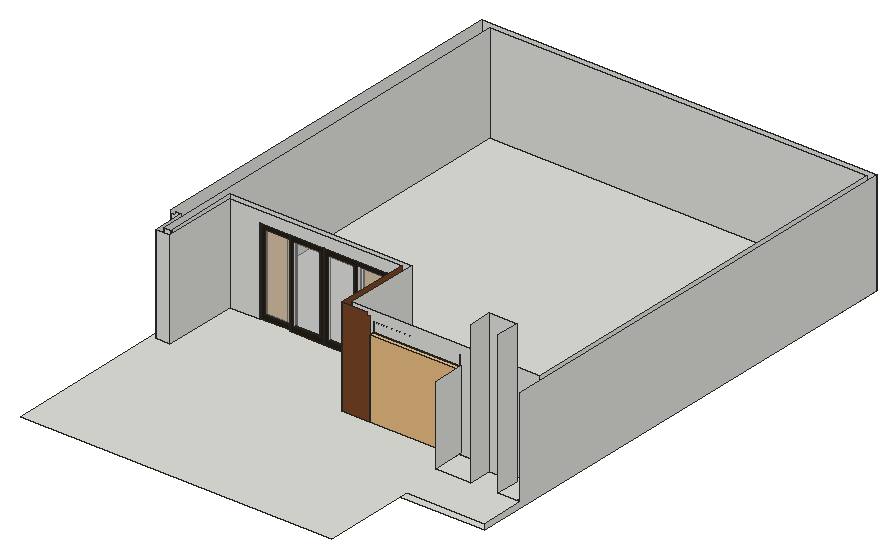
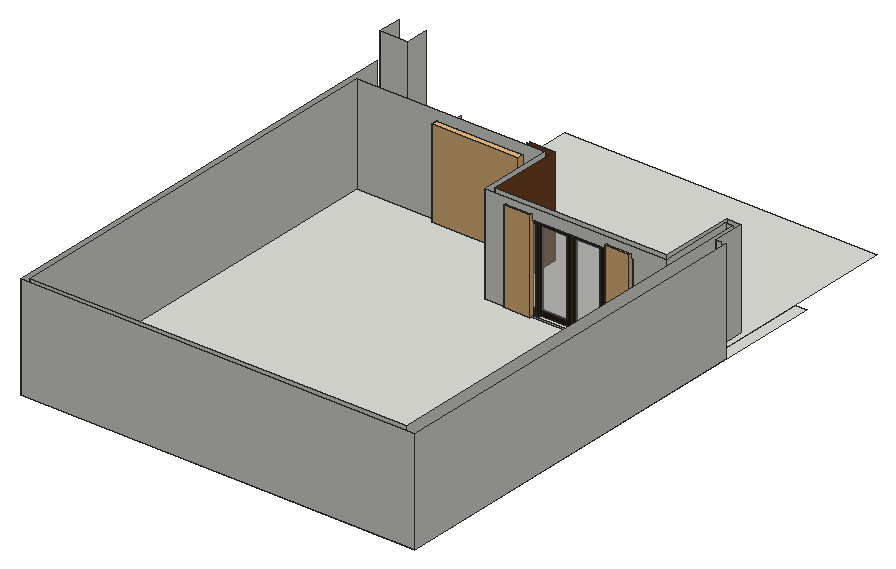
# SketchUp Ruby script. Lengths in inches.
U = 1.inch
M = Sketchup.active_model
def pt(a) = Geom::Point3d.new(a.map { |v| v * U })
def face(e, loops, mat)
  f = e.add_face(loops[0].map { |a| pt(a) })
  loops[1..].each { |l| e.add_face(l.map { |a| pt(a) }).erase! }
  f.material = f.back_material = mat if mat
  f
end
# faces: each face lists its corners as indices into pts; further lists are holes
def faces(e, pts, list, mat = nil) = list.each { |f| face(e, (f[0].is_a?(Array) ? f : [f]).map { |l| l.map { |i| pts[i] } }, mat) }
# xy, xz, yz: faces in a plane at the given z, y or x. An outline is a flat list of corners, or four numbers for a rectangle; further outlines are holes
def ring(l) = l.size == 4 ? [[l[0], l[1]], [l[2], l[1]], [l[2], l[3]], [l[0], l[3]]] : l.each_slice(2).to_a
def flat(e, list, mat, &to3) = list.each { |f| face(e, (f[0].is_a?(Array) ? f : [f]).map { |l| ring(l).map { |u, v| to3.(u, v) } }, mat) }
def xy(e, z, list, mat = nil) = flat(e, list, mat) { |x, y| [x, y, z] }
def xz(e, y, list, mat = nil) = flat(e, list, mat) { |x, z| [x, y, z] }
def yz(e, x, list, mat = nil) = flat(e, list, mat) { |y, z| [x, y, z] }
def lines(e, pts, list) = list.each { |a, b| e.add_line(pt(pts[a]), pt(pts[b])) }
# prism: a flat outline (further loops are holes) pulled along v
def prism(e, loops, v, mat = nil)
  f = face(e, loops, mat); d = Geom::Vector3d.new(v.map { |x| x * U })
  f.pushpull(f.normal.samedirection?(d) ? d.length : -d.length)
end
def box(e, o, s, mat = nil) = prism(e, [[o, [o[0] + s[0], o[1], o[2]], [o[0] + s[0], o[1] + s[1], o[2]], [o[0], o[1] + s[1], o[2]]]], [0, 0, s[2]], mat)
def at(x, y, z, deg = 0) = Geom::Transformation.translation(pt([x, y, z])) * Geom::Transformation.rotation(ORIGIN, Z_AXIS, deg.degrees)
def axes(o, x, y, z) = Geom::Transformation.new([*x, 0, *y, 0, *z, 0, *pt(o).to_a, 1])
def part(name) = M.definitions.add(name)
# library, detail: a bought-in or finely detailed component or shape, given as its bounding box
def library(name, o, s) = part(name).tap { |d| box(d.entities, o, s) }
def detail(e, o, s) = box(e.add_group.entities, o, s)
def put(e, d, t, mat = nil) = e.add_instance(d, t).tap { |i| i.material = mat if mat }
def group(e, t, mat = nil) = e.add_group.tap { |g| g.transformation = t; g.material = mat if mat }.entities
root = M.entities
M.materials.add("[Translucent Glass Gray]2").color = [201, 201, 201]
M.materials["[Translucent Glass Gray]2"].alpha = 0.5
M.materials.add("[Wood Veneer 01]").color = [120, 70, 37]
M.materials.add("curtain").color = [207, 207, 207]
M.materials["curtain"].alpha = 0.74
M.materials.add("oak swatch").color = [40, 31, 19]
c1 = library("Sliding Door",[0,0,0],[94.49,5.83,91.73])
c2 = library("Window curtains",[0,0,0],[5.91,79.92,51.3])
c3 = part("Group\#1")
box(c3.entities,[0,0,0],[1.77,4.72,80.31],"oak swatch")
c4 = part("Exterior Sliding Doors")
xy(c4.entities,0,[[1.77,33.07,3.54,70.87],[1.77,70.87,3.54,108.66]])
xy(c4.entities,0,[[0,0,1.77,33.07],[0,108.66,1.77,141.73]],"oak swatch")
xy(c4.entities,4.72,[[0,4.72,1.77,33.07],[1.77,37.8,3.54,66.14],[1.77,75.88,3.54,103.9375],[0,108.66,1.77,137.01]],"oak swatch")
xy(c4.entities,75.59,[[1.77,37.8,3.54,66.14],[1.77,75.88,3.54,103.9375]])
xy(c4.entities,75.59,[[0,4.72,1.77,33.07],[0,108.66,1.77,137.01]],"oak swatch")
xy(c4.entities,80.31,[[0,0,1.77,33.07],[1.77,33.07,3.54,70.87],[1.77,70.87,3.54,108.66],[0,108.66,1.77,141.73]],"oak swatch")
xz(c4.entities,0,[[0,0,1.77,80.31]],"oak swatch")
xz(c4.entities,4.72,[[0,4.72,1.77,75.59]],"oak swatch")
xz(c4.entities,33.07,[[0,0,1.77,4.72],[1.77,0,3.54,80.31],[0,75.59,1.77,80.31]],"oak swatch")
xz(c4.entities,37.8,[[1.77,4.72,3.54,75.59]])
xz(c4.entities,66.14,[[1.77,4.72,3.54,75.59]],"oak swatch")
xz(c4.entities,70.87,[[1.77,0,3.54,80.31]])
xz(c4.entities,75.88,[[1.77,4.72,3.54,75.59]])
xz(c4.entities,103.9375,[[1.77,4.72,3.54,75.59]],"oak swatch")
xz(c4.entities,108.66,[[1.77,4.72,3.54,75.59]])
xz(c4.entities,108.66,[[0,0,3.54,4.72],[0,75.59,3.54,80.31]],"oak swatch")
xz(c4.entities,137.01,[[0,4.72,1.77,75.59]],"oak swatch")
xz(c4.entities,141.73,[[0,0,1.77,80.31]],"oak swatch")
yz(c4.entities,0,[[0,0,33.07,0,33.07,4.72,4.72,4.72,4.72,75.59,33.07,75.59,33.07,80.31,0,80.31],[108.66,0,141.73,0,141.73,80.31,108.66,80.31,108.66,75.59,137.01,75.59,137.01,4.72,108.66,4.72]],"oak swatch")
yz(c4.entities,1.77,[[4.72,4.72,33.07,75.59],[37.8,4.72,66.14,75.59],[75.88,4.72,103.9375,75.59],[108.66,4.72,137.01,75.59]],"[Translucent Glass Gray]2")
yz(c4.entities,1.77,[[0,0,33.07,0,33.07,4.72,4.72,4.72,4.72,75.59,33.07,75.59,33.07,80.31,0,80.31],[[33.07,0,70.87,80.31],[37.8,4.72,66.14,75.59]],[[70.87,0,141.73,80.31],[108.66,4.72,137.01,75.59],[75.88,4.72,103.9375,75.59]]],"oak swatch")
yz(c4.entities,3.54,[[[33.07,0,70.87,80.31],[37.8,4.72,66.14,75.59]],[[70.87,0,108.66,80.31],[75.88,4.72,103.9375,75.59]]],"oak swatch")
put(c4.entities,c3,at(0,33.07,0))
put(c4.entities,c3,at(0,103.9375,0))
c5 = library("Plane02",[0.84,-3.92,-95.52],[32.2,7.84,95.63])
xy(root,252,[[177.75,508.37,177.75,1103.3125,657.75,1103.3125,657.75,508.37,431.89,508.37,431.89,692.93,220.5,692.93,220.5,721.37,447.875,721.37,447.875,522.1,645.31,522.1,645.31,1090.87,190.19,1090.87,190.19,508.37],[190.19,508.37,190.19,721.37,220.5,721.37,220.5,692.93,220.4375,692.93,220.4375,508.37],[[447.875,522.1,447.875,721.37,190.19,721.37,190.19,1090.87,645.31,1090.87,645.31,522.1],[380.99,855.03,382.54,855.24,383.99,855.84,385.23,856.79,386.1875,858.03,386.79,859.48,386.99,861.03,386.79,862.59,386.1875,864.03,385.23,865.28,383.99,866.23,382.54,866.83,380.99,867.03,379.4375,866.83,377.99,866.23,376.75,865.28,375.8,864.03,375.2,862.59,374.99,861.03,375.2,859.48,375.8,858.03,376.75,856.79,377.99,855.84,379.4375,855.24],[312.79,972.48,314.35,972.6875,315.79,973.29,317.04,974.24,317.99,975.48,318.59,976.93,318.79,978.48,318.59,980.04,317.99,981.48,317.04,982.72,315.79,983.68,314.35,984.28,312.79,984.48,311.24,984.28,309.79,983.68,308.55,982.72,307.6,981.48,307,980.04,306.79,978.48,307,976.93,307.6,975.48,308.55,974.24,309.79,973.29,311.24,972.6875],[380.99,920.01,382.54,920.22,383.99,920.81,385.23,921.77,386.1875,923.01,386.79,924.46,386.99,926.01,386.79,927.5625,386.1875,929.01,385.23,930.25,383.99,931.21,382.54,931.81,380.99,932.01,379.4375,931.81,377.99,931.21,376.75,930.25,375.8,929.01,375.2,927.5625,374.99,926.01,375.2,924.46,375.8,923.01,376.75,921.77,377.99,920.81,379.4375,920.22],[380.99,982.21,382.54,982.41,383.99,983.01,385.23,983.97,386.1875,985.21,386.79,986.66,386.99,988.21,386.79,989.76,386.1875,991.21,385.23,992.45,383.99,993.41,382.54,994.01,380.99,994.21,379.4375,994.01,377.99,993.41,376.75,992.45,375.8,991.21,375.2,989.76,374.99,988.21,375.2,986.66,375.8,985.21,376.75,983.97,377.99,983.01,379.4375,982.41],[312.79,900.05,314.04,900.21,315.2,900.7,316.2,901.46,316.97,902.46,317.45,903.62,317.61,904.87,317.45,906.11,316.97,907.28,316.2,908.27,315.2,909.04,314.04,909.52,312.79,909.68,311.55,909.52,310.39,909.04,309.39,908.27,308.62,907.28,308.14,906.11,307.98,904.87,308.14,903.62,308.62,902.46,309.39,901.46,310.39,900.7,311.55,900.21],[312.79,849.57,313.47,849.66,314.11,849.93,314.65,850.34,315.07,850.89,315.33,851.52,315.42,852.2,315.33,852.88,315.07,853.51,314.65,854.05,314.11,854.47,313.47,854.73,312.79,854.82,312.12,854.73,311.48,854.47,310.9375,854.05,310.52,853.51,310.26,852.88,310.17,852.2,310.26,851.52,310.52,850.89,310.9375,850.34,311.48,849.93,312.12,849.66]],[447.875,707.71,645.31,721.37]])
xy(root,253.1875,[[236.74,560.96,235.44,561.13,234.24,561.625,233.2,562.42,232.4,563.46,231.91,564.66,231.74,565.96,231.91,567.25,232.4,568.46,233.2,569.49,234.24,570.29,235.44,570.79,236.74,570.96,238.03,570.79,239.24,570.29,240.27,569.49,241.07,568.46,241.56,567.25,241.74,565.96,241.56,564.66,241.07,563.46,240.27,562.42,239.24,561.625,238.03,561.13]])
xy(root,258,[[193.12,600.32,201.88,600.32,201.88,690.57,422.81,690.57,422.81,600.32,651,600.32,651,1096.57,193.12,1096.57]])
xy(root,259.4375,[[183.75,394.64,562.6875,394.64,562.6875,508.37,657.75,508.37,657.75,562.125,631.02,562.125,631.02,589.625,597.99,589.625,597.99,562.125,554.88,562.125,554.88,600.32,449.19,600.32,449.19,593.57,416.0625,593.57,416.0625,683.82,398.4,683.82,398.4,690.57,243.65,690.57,243.65,683.82,206.9375,683.82,206.9375,593.57,189.75,593.57,189.75,631.27,183.75,631.27]])
xz(root,589.625,[[597.99,259.4375,631.02,431.7]])
xz(root,593.57,[[189.75,259.4375,206.9375,378]])
xz(root,593.57,[[416.0625,259.4375,449.19,259.4375,449.19,354.1875,449.43,354.1875,449.43,375.25,446,375.25,446,378,416.0625,378]],"[Wood Veneer 01]")
xz(root,600.32,[[193.12,258,201.88,378],[201.88,258,202.875,378],[422.81,258,422.81,378,651,378,651,258,554.88,258,554.88,354.1875,449.19,354.1875,449.19,258],[449.19,258,554.88,259.4375]])
xz(root,631.27,[[183.75,259.4375,189.75,259.4375,189.75,378,183.75,378,183.75,375.25,177.75,375.25,177.75,273.1875,183.75,273.1875]])
xz(root,683.82,[[206.9375,259.4375,243.65,259.4375,243.65,364.125,398.4,364.125,398.4,259.4375,416.0625,259.4375,416.0625,378,206.9375,378]])
xz(root,690.57,[[201.88,258,201.88,378,422.81,378,422.81,258,398.4,258,398.4,364.125,243.65,364.125,243.65,258],[243.65,258,398.4,259.4375]])
xz(root,1096.57,[[193.12,258,651,378]])
xz(root,1103.3125,[[177.75,252,657.75,378]])
yz(root,177.75,[[631.27,252,1103.3125,378]])
yz(root,189.75,[[593.57,259.4375,631.27,378]])
yz(root,193.12,[[600.32,258,1096.57,378]])
yz(root,201.88,[[600.32,258,690.57,378]])
yz(root,206.9375,[[593.57,259.4375,683.82,378]])
yz(root,243.65,[[683.82,259.4375,690.57,364.125]])
yz(root,398.4,[[683.82,259.4375,690.57,364.125]])
yz(root,416.0625,[[593.57,259.4375,683.82,378]],"[Wood Veneer 01]")
yz(root,422.81,[[600.32,258,690.57,378]])
yz(root,449.19,[[593.57,259.4375,600.32,354.1875]])
yz(root,554.88,[[562.125,259.4375,600.32,354.1875]])
yz(root,597.99,[[562.125,259.4375,589.625,431.7]])
yz(root,631.02,[[562.125,259.4375,589.625,431.7]])
yz(root,651,[[600.32,258,1096.57,378]])
yz(root,657.75,[[508.37,252,1103.3125,252,1103.3125,378,562.125,378,562.125,259.4375,508.37,259.4375]])
p = [[231.74,565.96,252],[231.91,567.25,252],[231.91,567.25,253.1875],[231.74,565.96,253.1875],[241.56,567.25,252],[241.74,565.96,252],
  [241.74,565.96,253.1875],[241.56,567.25,253.1875],[282.24,565.96,252],[282.41,567.25,252],[282.41,567.25,253.1875],[282.24,565.96,253.1875],
  [292.06,567.25,252],[292.24,565.96,252],[292.24,565.96,253.1875],[292.06,567.25,253.1875],[332.74,565.96,252],[332.91,567.25,252],
  [332.91,567.25,253.1875],[332.74,565.96,253.1875],[342.56,567.25,252],[342.74,565.96,252],[342.74,565.96,253.1875],[342.56,567.25,253.1875],
  [383.24,565.96,252],[383.41,567.25,252],[383.41,567.25,253.1875],[383.24,565.96,253.1875],[393.06,567.25,252],[393.24,565.96,252],
  [393.24,565.96,253.1875],[393.06,567.25,253.1875],[232.4,568.46,252],[232.4,568.46,253.1875],[241.07,568.46,252],[241.07,568.46,253.1875],
  [282.9,568.46,252],[282.9,568.46,253.1875],[291.57,568.46,252],[291.57,568.46,253.1875],[333.4,568.46,252],[333.4,568.46,253.1875],
  [342.07,568.46,252],[342.07,568.46,253.1875],[383.9,568.46,252],[383.9,568.46,253.1875],[392.57,568.46,252],[392.57,568.46,253.1875],
  [233.2,569.49,252],[233.2,569.49,253.1875],[240.27,569.49,252],[240.27,569.49,253.1875],[283.7,569.49,252],[283.7,569.49,253.1875],
  [290.77,569.49,252],[290.77,569.49,253.1875],[334.2,569.49,252],[334.2,569.49,253.1875],[341.27,569.49,252],[341.27,569.49,253.1875],
  [384.7,569.49,252],[384.7,569.49,253.1875],[391.77,569.49,252],[391.77,569.49,253.1875],[234.24,570.29,252],[234.24,570.29,253.1875],
  [239.24,570.29,252],[239.24,570.29,253.1875],[284.74,570.29,252],[284.74,570.29,253.1875],[289.74,570.29,252],[289.74,570.29,253.1875],
  [335.24,570.29,252],[335.24,570.29,253.1875],[340.24,570.29,252],[340.24,570.29,253.1875],[385.74,570.29,252],[385.74,570.29,253.1875],
  [390.74,570.29,252],[390.74,570.29,253.1875],[235.44,570.79,252],[235.44,570.79,253.1875],[238.03,570.79,252],[238.03,570.79,253.1875],
  [285.94,570.79,252],[285.94,570.79,253.1875],[288.53,570.79,252],[288.53,570.79,253.1875],[336.44,570.79,252],[336.44,570.79,253.1875],
  [339.03,570.79,252],[339.03,570.79,253.1875],[386.94,570.79,252],[386.94,570.79,253.1875],[389.53,570.79,252],[389.53,570.79,253.1875],
  [236.74,570.96,252],[236.74,570.96,253.1875],[287.24,570.96,252],[287.24,570.96,253.1875],[337.74,570.96,252],[337.74,570.96,253.1875],
  [388.24,570.96,252],[388.24,570.96,253.1875],[312.79,849.57,252],[312.12,849.66,252],[312.12,849.66,252.625],[312.79,849.57,252.625],
  [313.47,849.66,252],[313.47,849.66,252.625],[311.48,849.93,252],[311.48,849.93,252.625],[314.11,849.93,252],[314.11,849.93,252.625],
  [310.9375,850.34,252],[310.9375,850.34,252.625],[314.65,850.34,252],[314.65,850.34,252.625],[310.52,850.89,252],[310.52,850.89,252.625],
  [315.07,850.89,252],[315.07,850.89,252.625],[310.26,851.52,252],[310.26,851.52,252.625],[315.33,851.52,252],[315.33,851.52,252.625],
  [310.17,852.2,252],[310.17,852.2,252.625],[315.42,852.2,252],[315.42,852.2,252.625],[310.26,852.88,252],[310.26,852.88,252.625],
  [315.33,852.88,252],[315.33,852.88,252.625],[310.52,853.51,252],[310.52,853.51,252.625],[315.07,853.51,252],[315.07,853.51,252.625],
  [310.9375,854.05,252],[310.9375,854.05,252.625],[314.65,854.05,252],[314.65,854.05,252.625],[311.48,854.47,252],[311.48,854.47,252.625],
  [314.11,854.47,252],[314.11,854.47,252.625],[312.12,854.73,252],[312.12,854.73,252.625],[313.47,854.73,252],[313.47,854.73,252.625],
  [312.79,854.82,252],[312.79,854.82,252.625],[380.99,855.03,252],[379.4375,855.24,252],[379.4375,855.24,253.3125],[380.99,855.03,253.3125],
  [382.54,855.24,252],[382.54,855.24,253.3125],[377.99,855.84,252],[377.99,855.84,253.3125],[383.99,855.84,252],[383.99,855.84,253.3125],
  [376.75,856.79,252],[376.75,856.79,253.3125],[385.23,856.79,252],[385.23,856.79,253.3125],[375.8,858.03,252],[375.8,858.03,253.3125],
  [386.1875,858.03,252],[386.1875,858.03,253.3125],[375.2,859.48,252],[375.2,859.48,253.3125],[386.79,859.48,252],[386.79,859.48,253.3125],
  [374.99,861.03,252],[374.99,861.03,253.3125],[386.99,861.03,252],[386.99,861.03,253.3125],[375.2,862.59,252],[375.2,862.59,253.3125],
  [386.79,862.59,252],[386.79,862.59,253.3125],[375.8,864.03,252],[375.8,864.03,253.3125],[386.1875,864.03,252],[386.1875,864.03,253.3125],
  [376.75,865.28,252],[376.75,865.28,253.3125],[385.23,865.28,252],[385.23,865.28,253.3125],[377.99,866.23,252],[377.99,866.23,253.3125],
  [383.99,866.23,252],[383.99,866.23,253.3125],[379.4375,866.83,252],[379.4375,866.83,253.3125],[382.54,866.83,252],[382.54,866.83,253.3125],
  [380.99,867.03,252],[380.99,867.03,253.3125],[312.79,900.05,252],[311.55,900.21,252],[311.55,900.21,252.625],[312.79,900.05,252.625],
  [314.04,900.21,252],[314.04,900.21,252.625],[310.39,900.7,252],[310.39,900.7,252.625],[315.2,900.7,252],[315.2,900.7,252.625],
  [309.39,901.46,252],[309.39,901.46,252.625],[316.2,901.46,252],[316.2,901.46,252.625],[308.62,902.46,252],[308.62,902.46,252.625],
  [316.97,902.46,252],[316.97,902.46,252.625],[308.14,903.62,252],[308.14,903.62,252.625],[317.45,903.62,252],[317.45,903.62,252.625],
  [307.98,904.87,252],[307.98,904.87,252.625],[317.61,904.87,252],[317.61,904.87,252.625],[308.14,906.11,252],[308.14,906.11,252.625],
  [317.45,906.11,252],[317.45,906.11,252.625],[308.62,907.28,252],[308.62,907.28,252.625],[316.97,907.28,252],[316.97,907.28,252.625],
  [309.39,908.27,252],[309.39,908.27,252.625],[316.2,908.27,252],[316.2,908.27,252.625],[310.39,909.04,252],[310.39,909.04,252.625],
  [315.2,909.04,252],[315.2,909.04,252.625],[311.55,909.52,252],[311.55,909.52,252.625],[314.04,909.52,252],[314.04,909.52,252.625],
  [312.79,909.68,252],[312.79,909.68,252.625],[380.99,920.01,252],[379.4375,920.22,252],[379.4375,920.22,253.3125],[380.99,920.01,253.3125],
  [382.54,920.22,252],[382.54,920.22,253.3125],[377.99,920.81,252],[377.99,920.81,253.3125],[383.99,920.81,252],[383.99,920.81,253.3125],
  [376.75,921.77,252],[376.75,921.77,253.3125],[385.23,921.77,252],[385.23,921.77,253.3125],[375.8,923.01,252],[375.8,923.01,253.3125],
  [386.1875,923.01,252],[386.1875,923.01,253.3125],[375.2,924.46,252],[375.2,924.46,253.3125],[386.79,924.46,252],[386.79,924.46,253.3125],
  [374.99,926.01,252],[374.99,926.01,253.3125],[386.99,926.01,252],[386.99,926.01,253.3125],[375.2,927.5625,252],[375.2,927.5625,253.3125],
  [386.79,927.5625,252],[386.79,927.5625,253.3125],[375.8,929.01,252],[375.8,929.01,253.3125],[386.1875,929.01,252],[386.1875,929.01,253.3125],
  [376.75,930.25,252],[376.75,930.25,253.3125],[385.23,930.25,252],[385.23,930.25,253.3125],[377.99,931.21,252],[377.99,931.21,253.3125],
  [383.99,931.21,252],[383.99,931.21,253.3125],[379.4375,931.81,252],[379.4375,931.81,253.3125],[382.54,931.81,252],[382.54,931.81,253.3125],
  [380.99,932.01,252],[380.99,932.01,253.3125],[312.79,972.48,252],[311.24,972.6875,252],[311.24,972.6875,252.625],[312.79,972.48,252.625],
  [314.35,972.6875,252],[314.35,972.6875,252.625],[309.79,973.29,252],[309.79,973.29,252.625],[315.79,973.29,252],[315.79,973.29,252.625],
  [308.55,974.24,252],[308.55,974.24,252.625],[317.04,974.24,252],[317.04,974.24,252.625],[307.6,975.48,252],[307.6,975.48,252.625],
  [317.99,975.48,252],[317.99,975.48,252.625],[307,976.93,252],[307,976.93,252.625],[318.59,976.93,252],[318.59,976.93,252.625],
  [306.79,978.48,252],[306.79,978.48,252.625],[318.79,978.48,252],[318.79,978.48,252.625],[307,980.04,252],[307,980.04,252.625],
  [318.59,980.04,252],[318.59,980.04,252.625],[307.6,981.48,252],[307.6,981.48,252.625],[317.99,981.48,252],[317.99,981.48,252.625],
  [308.55,982.72,252],[308.55,982.72,252.625],[317.04,982.72,252],[317.04,982.72,252.625],[380.99,982.21,252],[379.4375,982.41,252],
  [379.4375,982.41,253.3125],[380.99,982.21,253.3125],[382.54,982.41,252],[382.54,982.41,253.3125],[377.99,983.01,252],[377.99,983.01,253.3125],
  [383.99,983.01,252],[383.99,983.01,253.3125],[309.79,983.68,252],[309.79,983.68,252.625],[315.79,983.68,252],[315.79,983.68,252.625],
  [376.75,983.97,252],[376.75,983.97,253.3125],[385.23,983.97,252],[385.23,983.97,253.3125],[311.24,984.28,252],[311.24,984.28,252.625],
  [314.35,984.28,252],[314.35,984.28,252.625],[375.8,985.21,252],[375.8,985.21,253.3125],[386.1875,985.21,252],[386.1875,985.21,253.3125],
  [312.79,984.48,252],[312.79,984.48,252.625],[375.2,986.66,252],[375.2,986.66,253.3125],[386.79,986.66,252],[386.79,986.66,253.3125],
  [374.99,988.21,252],[374.99,988.21,253.3125],[386.99,988.21,252],[386.99,988.21,253.3125],[375.2,989.76,252],[375.2,989.76,253.3125],
  [386.79,989.76,252],[386.79,989.76,253.3125],[375.8,991.21,252],[375.8,991.21,253.3125],[386.1875,991.21,252],[386.1875,991.21,253.3125],
  [376.75,992.45,252],[376.75,992.45,253.3125],[385.23,992.45,252],[385.23,992.45,253.3125],[377.99,993.41,252],[377.99,993.41,253.3125],
  [383.99,993.41,252],[383.99,993.41,253.3125],[379.4375,994.01,252],[379.4375,994.01,253.3125],[382.54,994.01,252],[382.54,994.01,253.3125],
  [380.99,994.21,252],[380.99,994.21,253.3125]]
faces(root,p,[[0,1,2,3],[4,5,6,7],[8,9,10,11],[12,13,14,15],[16,17,18,19],[20,21,22,23],[24,25,26,27],[28,29,30,31],
  [1,32,33,2],[34,4,7,35],[9,36,37,10],[38,12,15,39],[17,40,41,18],[42,20,23,43],[25,44,45,26],[46,28,31,47],
  [32,48,49,33],[50,34,35,51],[36,52,53,37],[54,38,39,55],[40,56,57,41],[58,42,43,59],[44,60,61,45],[62,46,47,63],
  [48,64,65,49],[66,50,51,67],[52,68,69,53],[70,54,55,71],[56,72,73,57],[74,58,59,75],[60,76,77,61],[78,62,63,79],
  [64,80,81,65],[82,66,67,83],[68,84,85,69],[86,70,71,87],[72,88,89,73],[90,74,75,91],[76,92,93,77],[94,78,79,95],
  [80,96,97,81],[96,82,83,97],[84,98,99,85],[98,86,87,99],[88,100,101,89],[100,90,91,101],[92,102,103,93],[102,94,95,103],
  [104,105,106,107],[108,104,107,109],[105,110,111,106],[112,108,109,113],[110,114,115,111],[116,112,113,117],[114,118,119,115],[120,116,117,121],
  [118,122,123,119],[124,120,121,125],[122,126,127,123],[128,124,125,129],[126,130,131,127],[132,128,129,133],[130,134,135,131],[136,132,133,137],
  [134,138,139,135],[140,136,137,141],[138,142,143,139],[144,140,141,145],[142,146,147,143],[148,144,145,149],[146,150,151,147],[150,148,149,151],
  [152,153,154,155],[156,152,155,157],[153,158,159,154],[160,156,157,161],[158,162,163,159],[164,160,161,165],[162,166,167,163],[168,164,165,169],
  [166,170,171,167],[172,168,169,173],[170,174,175,171],[176,172,173,177],[174,178,179,175],[180,176,177,181],[178,182,183,179],[184,180,181,185],
  [182,186,187,183],[188,184,185,189],[186,190,191,187],[192,188,189,193],[190,194,195,191],[196,192,193,197],[194,198,199,195],[198,196,197,199],
  [200,201,202,203],[204,200,203,205],[201,206,207,202],[208,204,205,209],[206,210,211,207],[212,208,209,213],[210,214,215,211],[216,212,213,217],
  [214,218,219,215],[220,216,217,221],[218,222,223,219],[224,220,221,225],[222,226,227,223],[228,224,225,229],[226,230,231,227],[232,228,229,233],
  [230,234,235,231],[236,232,233,237],[234,238,239,235],[240,236,237,241],[238,242,243,239],[244,240,241,245],[242,246,247,243],[246,244,245,247],
  [248,249,250,251],[252,248,251,253],[249,254,255,250],[256,252,253,257],[254,258,259,255],[260,256,257,261],[258,262,263,259],[264,260,261,265],
  [262,266,267,263],[268,264,265,269],[266,270,271,267],[272,268,269,273],[270,274,275,271],[276,272,273,277],[274,278,279,275],[280,276,277,281],
  [278,282,283,279],[284,280,281,285],[282,286,287,283],[288,284,285,289],[286,290,291,287],[292,288,289,293],[290,294,295,291],[294,292,293,295],
  [296,297,298,299],[300,296,299,301],[297,302,303,298],[304,300,301,305],[302,306,307,303],[308,304,305,309],[306,310,311,307],[312,308,309,313],
  [310,314,315,311],[316,312,313,317],[314,318,319,315],[320,316,317,321],[318,322,323,319],[324,320,321,325],[322,326,327,323],[328,324,325,329],
  [326,330,331,327],[332,328,329,333],[334,335,336,337],[338,334,337,339],[335,340,341,336],[342,338,339,343],[330,344,345,331],[346,332,333,347],
  [340,348,349,341],[350,342,343,351],[344,352,353,345],[354,346,347,355],[348,356,357,349],[358,350,351,359],[352,360,361,353],[360,354,355,361],
  [356,362,363,357],[364,358,359,365],[362,366,367,363],[368,364,365,369],[366,370,371,367],[372,368,369,373],[370,374,375,371],[376,372,373,377],
  [374,378,379,375],[380,376,377,381],[378,382,383,379],[384,380,381,385],[382,386,387,383],[388,384,385,389],[386,390,391,387],[390,388,389,391]])
put(root,c1,axes([449.05,593.57,259.4375],[1.12,0,0],[0,1,0],[0,0,1.0329]))
put(root,c2,axes([553.89,600.32,259.5],[0,1.31,0],[-1.31,0,0],[0,0,2.07462]))
put(root,c4,axes([243.65,687.72,259.4375],[0,-1.1,0],[1.1,0,0],[0,0,1.30346]))
put(root,c5,axes([275.15,690.77,369.32],[-0.88913,0,0],[0,0.67314,0],[0,0,1.16538]),"curtain")
put(root,c5,axes([398.6875,690.77,369.79],[-0.97301,0,0],[0,0.67314,0],[0,0,1.16538]),"curtain")
g1 = group(root,at(306.79,849.57,252.625))
xy(g1,0,[[6,0,5.32,0.09,4.6875,0.35,4.14,0.77,3.73,1.3125,3.46,1.95,3.375,2.625,3.46,3.3,3.73,3.9375,4.14,4.48,4.6875,4.9,5.32,5.16,6,5.25,6.68,5.16,7.3125,4.9,7.86,4.48,8.27,3.9375,8.54,3.3,8.625,2.625,8.54,1.95,8.27,1.3125,7.86,0.77,7.3125,0.35,6.68,0.09],[6,50.48,4.75,50.64,3.59,51.12,2.59,51.89,1.83,52.88,1.35,54.05,1.18,55.29,1.35,56.54,1.83,57.7,2.59,58.7,3.59,59.47,4.75,59.95,6,60.11,7.25,59.95,8.41,59.47,9.41,58.7,10.17,57.7,10.65,56.54,10.82,55.29,10.65,54.05,10.17,52.88,9.41,51.89,8.41,51.12,7.25,50.64],[6,122.91,4.45,123.11,3,123.71,1.76,124.67,0.8,125.91,0.2,127.36,0,128.91,0.2,130.46,0.8,131.91,1.76,133.15,3,134.1,4.45,134.7,6,134.91,7.55,134.7,9,134.1,10.24,133.15,11.2,131.91,11.8,130.46,12,128.91,11.8,127.36,11.2,125.91,10.24,124.67,9,123.71,7.55,123.11]])
g2 = group(root,at(374.99,855.03,253.3125))
xy(g2,0,[[6,0,4.45,0.2,3,0.8,1.76,1.76,0.8,3,0.2,4.45,0,6,0.2,7.55,0.8,9,1.76,10.24,3,11.2,4.45,11.8,6,12,7.55,11.8,9,11.2,10.24,10.24,11.2,9,11.8,7.55,12,6,11.8,4.45,11.2,3,10.24,1.76,9,0.8,7.55,0.2],[6,64.98,4.45,65.18,3,65.78,1.76,66.73,0.8,67.98,0.2,69.42,0,70.98,0.2,72.53,0.8,73.98,1.76,75.22,3,76.17,4.45,76.77,6,76.98,7.55,76.77,9,76.17,10.24,75.22,11.2,73.98,11.8,72.53,12,70.98,11.8,69.42,11.2,67.98,10.24,66.73,9,65.78,7.55,65.18],[6,127.17,4.45,127.38,3,127.98,1.76,128.93,0.8,130.17,0.2,131.62,0,133.17,0.2,134.73,0.8,136.17,1.76,137.42,3,138.37,4.45,138.97,6,139.17,7.55,138.97,9,138.37,10.24,137.42,11.2,136.17,11.8,134.73,12,133.17,11.8,131.62,11.2,130.17,10.24,128.93,9,127.98,7.55,127.38]])
